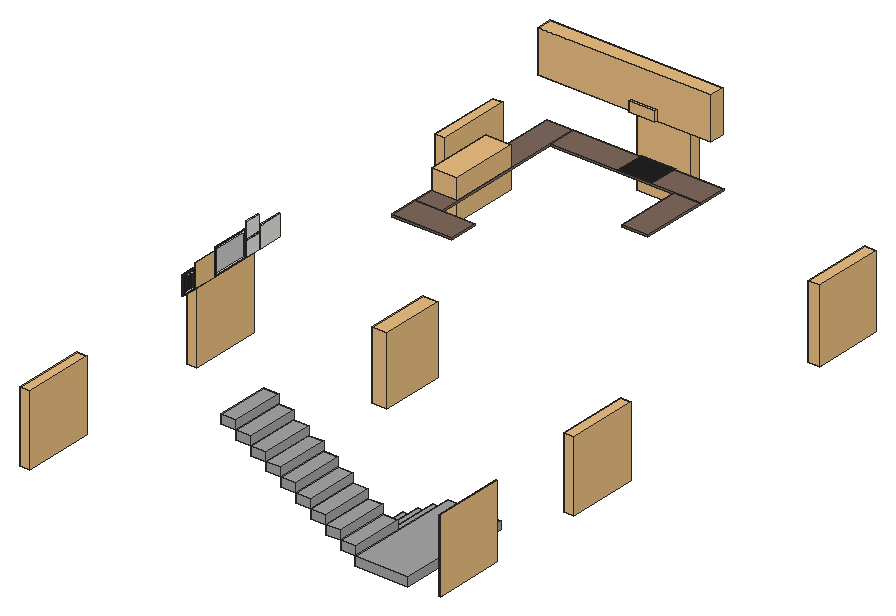
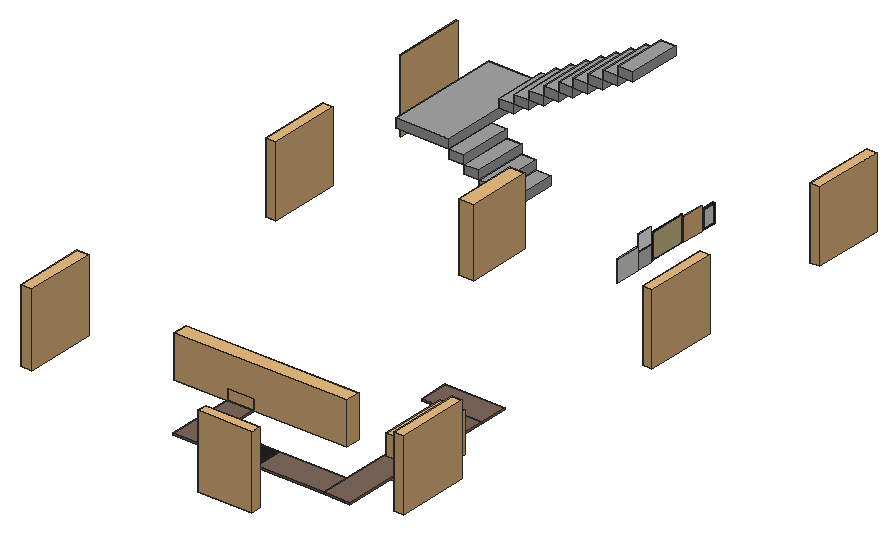
# SketchUp Ruby script. Lengths in inches.
U = 1.inch
M = Sketchup.active_model
def pt(a) = Geom::Point3d.new(a.map { |v| v * U })
def face(e, loops, mat)
  f = e.add_face(loops[0].map { |a| pt(a) })
  loops[1..].each { |l| e.add_face(l.map { |a| pt(a) }).erase! }
  f.material = f.back_material = mat if mat
  f
end
# faces: each face lists its corners as indices into pts; further lists are holes
def faces(e, pts, list, mat = nil) = list.each { |f| face(e, (f[0].is_a?(Array) ? f : [f]).map { |l| l.map { |i| pts[i] } }, mat) }
# xy, xz, yz: faces in a plane at the given z, y or x. An outline is a flat list of corners, or four numbers for a rectangle; further outlines are holes
def ring(l) = l.size == 4 ? [[l[0], l[1]], [l[2], l[1]], [l[2], l[3]], [l[0], l[3]]] : l.each_slice(2).to_a
def flat(e, list, mat, &to3) = list.each { |f| face(e, (f[0].is_a?(Array) ? f : [f]).map { |l| ring(l).map { |u, v| to3.(u, v) } }, mat) }
def xy(e, z, list, mat = nil) = flat(e, list, mat) { |x, y| [x, y, z] }
def xz(e, y, list, mat = nil) = flat(e, list, mat) { |x, z| [x, y, z] }
def yz(e, x, list, mat = nil) = flat(e, list, mat) { |y, z| [x, y, z] }
def lines(e, pts, list) = list.each { |a, b| e.add_line(pt(pts[a]), pt(pts[b])) }
# prism: a flat outline (further loops are holes) pulled along v
def prism(e, loops, v, mat = nil)
  f = face(e, loops, mat); d = Geom::Vector3d.new(v.map { |x| x * U })
  f.pushpull(f.normal.samedirection?(d) ? d.length : -d.length)
end
def box(e, o, s, mat = nil) = prism(e, [[o, [o[0] + s[0], o[1], o[2]], [o[0] + s[0], o[1] + s[1], o[2]], [o[0], o[1] + s[1], o[2]]]], [0, 0, s[2]], mat)
def at(x, y, z, deg = 0) = Geom::Transformation.translation(pt([x, y, z])) * Geom::Transformation.rotation(ORIGIN, Z_AXIS, deg.degrees)
def axes(o, x, y, z) = Geom::Transformation.new([*x, 0, *y, 0, *z, 0, *pt(o).to_a, 1])
def part(name) = M.definitions.add(name)
# library, detail: a bought-in or finely detailed component or shape, given as its bounding box
def library(name, o, s) = part(name).tap { |d| box(d.entities, o, s) }
def detail(e, o, s) = box(e.add_group.entities, o, s)
def put(e, d, t, mat = nil) = e.add_instance(d, t).tap { |i| i.material = mat if mat }
def group(e, t, mat = nil) = e.add_group.tap { |g| g.transformation = t; g.material = mat if mat }.entities
root = M.entities
M.materials.add("1 (6)").color = [39, 39, 39]
M.materials.add("2").color = [201, 201, 201]
M.materials.add("3").color = [255, 255, 255]
M.materials.add("5").color = [30, 30, 30]
M.materials.add("6").color = [210, 193, 141]
M.materials.add("Sophie_Hair1").color = [198, 198, 198]
M.materials.add("Sophie_Hair2").color = [255, 255, 255]
M.materials.add("Steve_Hair1").color = [228, 228, 225]
M.materials.add("[0136_Charcoal]").color = [34, 34, 34]
M.materials.add("[Color_008]1").color = [30, 30, 30]
M.materials.add("[Granite Brown]").color = [126, 104, 91]
M.materials.add("[Stone Vein Gray]").color = [166, 165, 165]
M.materials.add("[White Square Tile]").color = [33, 33, 33]
M.materials.add("cover").color = [255, 255, 255]
c1 = part("Group\#5")
box(c1.entities,[0,0,0],[10.125,36,6])
c2 = library("Group\#67",[0.125,0,0],[4,104,82])
c3 = library("KITCHEN SINK ",[0,0,-7.53],[55.12,22.64,27.32])
c4 = library("Agrupar\#2",[0,-7.38,0],[12.4,73.82,70.87])
c5 = part("Группа\#47")
xy(c5.entities,0,[[0,0,23.31,20.55]],"[0136_Charcoal]")
xy(c5.entities,0.2,[[0.36,0.64,22.93,20.59]],"[White Square Tile]")
p = [[0.36,20.13,0.2],[0.36,0.64,0.2],[0,0,0],[0,20.55,0],[0.36,20.59,0.2],[22.93,0.64,0.2],
  [23.31,0,0],[23.31,20.55,0],[22.93,20.13,0.2],[22.93,20.5625,0.2],[22.93,20.59,0.2]]
faces(c5.entities,p,[[0,1,2,3,4],[1,5,6,2],[7,6,5,8,9,10],[3,7,10,4]],"[0136_Charcoal]")
c6 = library("QUADRO-PAINTING",[182.91,225.91,15.99],[37.91,1.95,39.37])
c7 = part("Agrupar\#33")
xy(c7.entities,5.15,[[0,0,45.82,0.79]],"5")
xy(c7.entities,5.9375,[[0.79,0.39,45.03,0.55]],"3")
xy(c7.entities,5.9375,[[0.79,0.2,45.03,0.39],[0.79,0.55,45.03,0.79]],"5")
xy(c7.entities,7.12,[[1.97,0.39,43.85,0.47]],"3")
xy(c7.entities,35.04,[[1.97,0.39,43.85,0.47]],"3")
xy(c7.entities,36.22,[[0.79,0.39,45.03,0.55]],"3")
xy(c7.entities,36.22,[[0.79,0.2,45.03,0.39],[0.79,0.55,45.03,0.79]],"5")
xy(c7.entities,37.01,[[0,0,45.82,0.79]],"5")
xz(c7.entities,0.39,[[[0.79,5.9375,45.03,36.22],[1.97,7.12,43.85,35.04]]],"3")
xz(c7.entities,0.47,[[1.97,7.12,43.85,35.04]],"2")
xz(c7.entities,0.55,[[[0.79,5.9375,45.03,36.22],[1.97,7.12,43.85,35.04]]],"3")
xz(c7.entities,0.79,[[0,5.15,0,37.01,0.79,36.22,0.79,5.9375],[0,5.15,0.79,5.9375,45.03,5.9375,45.82,5.15],[45.82,5.15,45.03,5.9375,45.03,36.22,45.82,37.01],[0.79,36.22,0,37.01,45.82,37.01,45.03,36.22]],"5")
yz(c7.entities,0,[[0,5.15,0.79,37.01]],"5")
yz(c7.entities,0.79,[[0.39,5.9375,0.55,36.22]],"3")
yz(c7.entities,0.79,[[0.2,5.9375,0.39,36.22],[0.55,5.9375,0.79,36.22]],"5")
yz(c7.entities,1.97,[[0.39,7.12,0.47,35.04]],"3")
yz(c7.entities,43.85,[[0.39,7.12,0.47,35.04]],"3")
yz(c7.entities,45.03,[[0.39,5.9375,0.55,36.22]],"3")
yz(c7.entities,45.03,[[0.2,5.9375,0.39,36.22],[0.55,5.9375,0.79,36.22]],"5")
yz(c7.entities,45.82,[[0,5.15,0.79,37.01]],"5")
p = [[0,0,5.15],[0.79,0.2,5.9375],[0.79,0.2,36.22],[0,0,37.01],[45.82,0,5.15],[45.03,0.2,5.9375],
  [0.79,0.79,5.9375],[0,0.79,5.15],[0.79,0.39,5.9375],[0.79,0.55,5.9375],[45.82,0,37.01],[45.03,0.2,36.22],
  [45.82,0.79,5.15],[45.03,0.79,5.9375],[45.03,0.55,5.9375],[45.03,0.39,5.9375],[0,0.79,37.01],[0.79,0.79,36.22],
  [0.79,0.55,36.22],[0.79,0.39,36.22],[45.03,0.79,36.22],[45.82,0.79,37.01],[45.03,0.39,36.22],[45.03,0.55,36.22],
  [1.97,0.55,35.04],[1.97,0.47,35.04],[43.85,0.55,35.04],[43.85,0.47,35.04],[1.97,0.55,7.12],[1.97,0.47,7.12],
  [43.85,0.55,7.12],[43.85,0.47,7.12]]
faces(c7.entities,p,[[0,1,2,3],[4,5,1,0],[4,10,11,5],[11,10,3,2]],"5")
faces(c7.entities,p,[[6,7,0,1,8,9],[12,13,14,15,5,4],[16,17,18,19,2,3],[20,21,10,11,22,23]])
lines(c7.entities,p,[[24,25],[26,27],[28,29],[30,31]])
c8 = part("Agrupar\#32")
xz(c8.entities,0,[[0,0,62.39,42.7]],"6")
c9 = part("Agrupar\#34")
put(c9.entities,c7,axes([0,0,-7.26],[1.41,0,0],[0,1.41,0],[0,0,1.41]))
put(c9.entities,c8,at(1.11,0.86,1.11))
c10 = part("quadro_morozini (1)")
put(c10.entities,c9,at(0,0,0))
c11 = part("TY004BG-B8686")
g1 = group(c11.entities,at(80,43.32,0))
xy(g1,0,[[0,0,33.86,2.36]],"Sophie_Hair1")
xy(g1,33.86,[[0,0,33.86,2.36]],"Sophie_Hair1")
xz(g1,0,[[0,0,33.86,33.86]])
xz(g1,2.36,[[0,0,33.86,33.86]],"Sophie_Hair1")
yz(g1,0,[[0,0,2.36,33.86]],"Sophie_Hair1")
yz(g1,33.86,[[0,0,2.36,33.86]],"Sophie_Hair1")
c12 = part("Agrupar\#36")
prism(c12.entities,[[[9.45,12.875,-0.1],[9.45,0,-0.1],[0,0,-0.1],[0,12.875,-0.1]],[[8.86,0.59,-0.1],[8.86,12.28,-0.1],[0.59,12.28,-0.1],[0.59,0.59,-0.1]]],[0,0,0.39],"[Color_008]1")
c13 = part("Agrupar\#35")
xy(c13.entities,0,[[0,0,8.27,11.69]])
xy(c13.entities,0.1,[[0.79,0.79,7.48,10.91]],"1 (6)")
xy(c13.entities,0.1,[[[0,0,8.27,11.69],[0.79,0.79,7.48,10.91]]],"cover")
xz(c13.entities,0,[[0,0,8.27,0.1]])
xz(c13.entities,11.69,[[0,0,8.27,0.1]])
yz(c13.entities,0,[[0,0,11.69,0.1]])
yz(c13.entities,8.27,[[0,0,11.69,0.1]])
c14 = part("Agrupar\#37")
put(c14.entities,c12,at(0,0,0.1))
put(c14.entities,c13,at(0.59,0.59,0.1))
c15 = library("Group\#92",[0,0,0],[153.54,12.32,28.39])
c16 = library("Golden Vantage GURR136 - 36\" Under Cabinet Kitchen Range Hoo",[-17.91,-10.24,-10.09],[35.82,22.52,10.09])
c17 = part("LN093B-967")
g2 = group(c17.entities,at(80,43.32,0))
xy(g2,0,[[0,0,31.89,2.36]],"Sophie_Hair2")
xy(g2,32.28,[[0,0,31.89,2.36]],"Sophie_Hair2")
xz(g2,0,[[0,0,31.89,32.28]])
xz(g2,2.36,[[0,0,31.89,32.28]],"Sophie_Hair2")
yz(g2,0,[[0,0,2.36,32.28]],"Sophie_Hair2")
yz(g2,31.89,[[0,0,2.36,32.28]],"Sophie_Hair2")
put(root,c1,at(178.5,130,24),"[Stone Vein Gray]")
put(root,c1,at(188.625,130,30),"[Stone Vein Gray]")
put(root,c2,axes([-0.21,219,36],[1.67,0,0],[0,0.46827,0],[0,0,0.58537]))
put(root,c2,axes([-0.21,78,36],[1.67,0,0],[0,0.46154,0],[0,0,0.58537]))
put(root,c1,at(198.75,130,36),"[Stone Vein Gray]")
put(root,c2,axes([105,514.25,36],[0,1.67,0],[-0.35,0,0],[0,0,0.6]))
put(root,c2,axes([254.76,426,36],[1.9539,0,0],[0,0.46154,0],[0,0,0.6]))
put(root,c2,axes([255,219,36],[1.67,0,0],[0,0.46154,0],[0,0,0.58537]))
put(root,c2,axes([260.16,107,36],[0.2839,0,0],[0,0.46154,0],[0,0,0.6]))
put(root,c2,axes([2.11,426,37.625],[1.67,0,0],[0,0.469,0],[0,0,0.58537]))
put(root,c1,at(208.875,130,42),"[Stone Vein Gray]")
put(root,c3,axes([26.1875,414.625,52.52],[0,0.8316,0.00001],[-0.75918,0,0.00001],[0.00001,-0.00001,1]),"Steve_Hair1")
g3 = group(root,at(219,130,48),"[Stone Vein Gray]")
box(g3,[0,-42.4375,0],[36,78.4375,6])
put(root,c4,axes([128.31,267.06,49.7],[-0.832,0,0],[0,-0.5876,0],[0,0,0.65]))
put(root,c1,at(208.875,88,54),"[Stone Vein Gray]")
g4 = group(root,at(9.18,381,57.73),"[Granite Brown]")
g5 = group(g4,at(0,19.64,0))
xy(g5,0,[[[0,0,17.93,111.32],[3.63,15.7,15.44,43.37]]])
xy(g5,1.18,[[[0,0,17.93,111.32],[3.57,15.63,15.5,43.43]]],"[Granite Brown]")
xz(g5,0,[[0,0,17.93,1.18]])
xz(g5,111.32,[[0,0,17.93,1.18]])
yz(g5,0,[[0,0,111.32,1.18]])
yz(g5,17.93,[[0,0,111.32,1.18]])
p = [[3.63,15.7,1.18],[3.63,15.7,0],[15.5,15.63,0],[15.5,15.63,1.18]]
faces(g5,p,[[0,1,2,3]])
g6 = group(g4,at(17.93,111.32,0))
xy(g6,0,[[0,0,101.89,19.64]])
xy(g6,1.18,[[0,0,101.89,19.64]],"[Granite Brown]")
xz(g6,0,[[0,0,101.89,1.18]])
xz(g6,19.64,[[0,0,101.89,1.18]])
yz(g6,0,[[0,0,19.64,1.18]])
yz(g6,101.89,[[0,0,19.64,1.18]])
g7 = group(g4,at(101.89,67.12,0))
box(g7,[0,0,0],[17.93,44.2,1.18])
g8 = group(g4,at(0,0,0))
xy(g8,0,[[0,0,40.35,19.64]])
xy(g8,1.18,[[0,0,40.35,19.64]],"[Granite Brown]")
xz(g8,0,[[0,0,0.27,1.18],[0.27,0,40.35,1.18]])
xz(g8,19.64,[[0,0,40.35,1.18]])
yz(g8,0,[[0,0,19.64,1.18]])
yz(g8,40.35,[[0,0,19.64,1.18]])
put(root,c5,at(72.43,492.32,58.91))
put(root,c1,at(198.75,88,60),"[Stone Vein Gray]")
put(root,c1,at(188.625,88,66),"[Stone Vein Gray]")
put(root,c1,at(178.5,88,72),"[Stone Vein Gray]")
put(root,c1,at(168.375,88,78),"[Stone Vein Gray]")
put(root,c1,at(158.25,88,84),"[Stone Vein Gray]")
put(root,c1,at(148.125,88,90),"[Stone Vein Gray]")
put(root,c6,axes([100.93,139.36,83.86],[0,0.39,0],[-0.39,0,0],[0,0,0.39]))
put(root,c10,axes([12.83,227.01,90.11],[0,0.39,0],[-0.39,0,0],[0,0,0.39]))
put(root,c11,axes([28.04,230.14,90.11],[0,0.29504,0],[-0.34961,0,0],[0,0,0.29504]))
g9 = group(root,at(12.71,265.27,90.11))
box(g9,[-0.83,0,0],[0.83,16.43,14.1])
put(root,c14,axes([12.07,199.95,90.11],[0,0.975,0],[0,0,0.975],[2.89182,0,0]))
put(root,c15,axes([11.6875,501.71,91.61],[0.75918,0,0],[0,0.8316,0],[0,0,1]),"Steve_Hair1")
put(root,c16,axes([83.37,505.27,98.74],[0.49764,0,0],[0,0.54511,0],[0,0,0.6555]),"Steve_Hair1")
put(root,c1,at(138,88,96),"[Stone Vein Gray]")
put(root,c17,axes([28.04,228.68,101.46],[0,0.31325,0],[-0.34961,0,0],[0,0,0.31239]))
g10 = group(root,at(127.875,88,102),"[Stone Vein Gray]")
box(g10,[0,0,0],[10.125,36,6])
